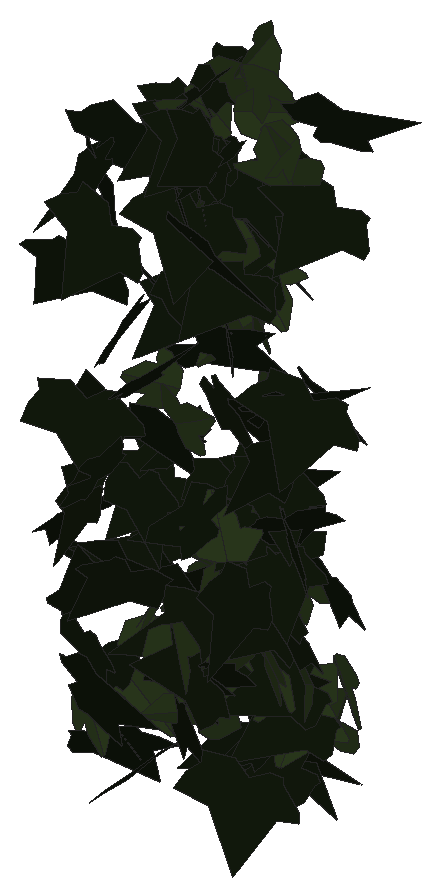
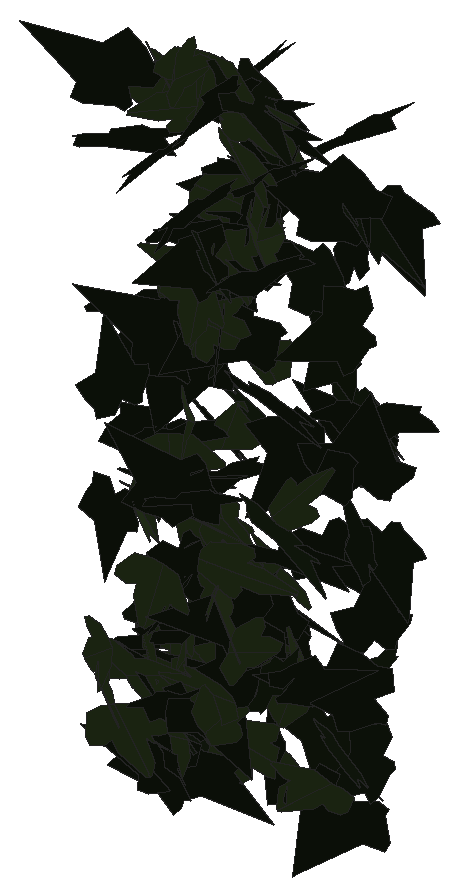
# SketchUp Ruby script. Lengths in inches.
U = 1.inch
M = Sketchup.active_model
def pt(a) = Geom::Point3d.new(a.map { |v| v * U })
def face(e, loops, mat)
  f = e.add_face(loops[0].map { |a| pt(a) })
  loops[1..].each { |l| e.add_face(l.map { |a| pt(a) }).erase! }
  f.material = f.back_material = mat if mat
  f
end
# faces: each face lists its corners as indices into pts; further lists are holes
def faces(e, pts, list, mat = nil) = list.each { |f| face(e, (f[0].is_a?(Array) ? f : [f]).map { |l| l.map { |i| pts[i] } }, mat) }
# xy, xz, yz: faces in a plane at the given z, y or x. An outline is a flat list of corners, or four numbers for a rectangle; further outlines are holes
def ring(l) = l.size == 4 ? [[l[0], l[1]], [l[2], l[1]], [l[2], l[3]], [l[0], l[3]]] : l.each_slice(2).to_a
def flat(e, list, mat, &to3) = list.each { |f| face(e, (f[0].is_a?(Array) ? f : [f]).map { |l| ring(l).map { |u, v| to3.(u, v) } }, mat) }
def xy(e, z, list, mat = nil) = flat(e, list, mat) { |x, y| [x, y, z] }
def xz(e, y, list, mat = nil) = flat(e, list, mat) { |x, z| [x, y, z] }
def yz(e, x, list, mat = nil) = flat(e, list, mat) { |y, z| [x, y, z] }
def lines(e, pts, list) = list.each { |a, b| e.add_line(pt(pts[a]), pt(pts[b])) }
# prism: a flat outline (further loops are holes) pulled along v
def prism(e, loops, v, mat = nil)
  f = face(e, loops, mat); d = Geom::Vector3d.new(v.map { |x| x * U })
  f.pushpull(f.normal.samedirection?(d) ? d.length : -d.length)
end
def box(e, o, s, mat = nil) = prism(e, [[o, [o[0] + s[0], o[1], o[2]], [o[0] + s[0], o[1] + s[1], o[2]], [o[0], o[1] + s[1], o[2]]]], [0, 0, s[2]], mat)
def at(x, y, z, deg = 0) = Geom::Transformation.translation(pt([x, y, z])) * Geom::Transformation.rotation(ORIGIN, Z_AXIS, deg.degrees)
def axes(o, x, y, z) = Geom::Transformation.new([*x, 0, *y, 0, *z, 0, *pt(o).to_a, 1])
def part(name) = M.definitions.add(name)
# library, detail: a bought-in or finely detailed component or shape, given as its bounding box
def library(name, o, s) = part(name).tap { |d| box(d.entities, o, s) }
def detail(e, o, s) = box(e.add_group.entities, o, s)
def put(e, d, t, mat = nil) = e.add_instance(d, t).tap { |i| i.material = mat if mat }
def group(e, t, mat = nil) = e.add_group.tap { |g| g.transformation = t; g.material = mat if mat }.entities
root = M.entities
M.materials.add("1026 AP 7946 SUNNY SIDE UP").color = [254, 231, 186]
M.materials.add("efeu1").color = [18, 25, 13]
M.materials.add("efeu2").color = [43, 57, 29]
c1 = part("ivyleaf_9")
p = [[1.54,2.16,1.25],[1.36,2.04,1.19],[-0.21,0.99,0.68],[-0.71,1.11,0.82],[-0.85,0.86,0.67],[-0.8,0.17,0.21],
  [-0.9,-0.01,0.1],[-0.67,-0.16,-0.02],[-0.08,-0.08,-0.05],[-0.03,-0.6,-0.4],[0.65,-0.88,-0.66],[0.83,-0.6,-0.49],
  [1.29,-0.42,-0.43],[1.8125,-0.07,-0.26],[1.21,0.44,0.15]]
faces(c1.entities,p,[[0,1,2,3,4,5,6,7,8,9,10,11,12,13,14]],"efeu1")
c2 = part("ivyleaf_10")
p = [[0,0.5,-0.03],[-0.0625,2.02,-0.43],[-0.19,2.01,-0.46],[-0.54,1.05,-0.29],[-0.52,0.625,-0.18],[-0.83,0.76,-0.28],
  [-1.16,0.64,-0.33],[-1.15,0.33,-0.24],[-0.77,-0.39,0.02],[-0.3,-0.51,0.16],[0.04,-0.48,0.23],[-0.02,2.01,-0.4375],
  [-0.06,2.01,-0.43],[0.04,-0.49,0.23],[0.67,-0.49,0.14],[1.38,0.36,-0.2],[1.375,0.51,-0.24],[0.81,0.65,-0.19],
  [0.62,0.59,-0.15],[0.6,1.09,-0.28],[0.5,1.23,-0.31]]
faces(c2.entities,p,[[0,1,2,3,4,5,6,7,8,9,10],[11,12,0,13,14,15,16,17,18,19,20]],"efeu2")
put(root,c1,axes([143.12,206.38,282.79],[0.44243,-0.08398,-0.36172],[0.56659,0.04987,0.28587],[-0.01992,-0.4468,0.09716]),"1026 AP 7946 SUNNY SIDE UP")
put(root,c1,axes([142.05,208.34,288.9],[-0.2726,-0.37462,0.23144],[-0.11476,-0.21578,-0.42595],[0.67895,-0.18688,0.02093]),"1026 AP 7946 SUNNY SIDE UP")
put(root,c1,axes([141.82,208.15,284.62],[-0.4204,0.06283,-0.26024],[0.35853,-0.11923,-0.27946],[-0.1986,-0.34823,0.04639]),"1026 AP 7946 SUNNY SIDE UP")
put(root,c1,axes([144.47,208.41,283.86],[-0.56265,0.0144,-0.29484],[0.43446,-0.10455,-0.36181],[-0.11997,-0.44617,0.07251]),"1026 AP 7946 SUNNY SIDE UP")
put(root,c1,axes([141.93,208.21,284.87],[-0.15575,0.37355,0.17332],[-0.08965,0.15663,-0.39696],[-0.63655,-0.11346,0.0135]),"1026 AP 7946 SUNNY SIDE UP")
put(root,c1,axes([141.4375,208.46,288.125],[0.29042,0.15248,-0.34098],[-0.36608,-0.23735,-0.24723],[-0.44243,0.29648,-0.01926]),"1026 AP 7946 SUNNY SIDE UP")
put(root,c1,axes([142.39,208.34,286.4],[0.14354,0.3645,0.012],[-0.01735,-0.00711,0.38695],[0.57307,-0.09152,0.00871]),"1026 AP 7946 SUNNY SIDE UP")
put(root,c1,axes([143.16,209.09,281.73],[0.15178,-0.38666,-0.21939],[0.10483,-0.20045,0.40912],[-0.68446,-0.11644,0.01401]),"1026 AP 7946 SUNNY SIDE UP")
put(root,c2,axes([141.36,208.77,280.88],[0.07741,0.38036,0.01188],[0.01152,0.0085,-0.39501],[-0.59815,0.04939,-0.00607]),"1026 AP 7946 SUNNY SIDE UP")
put(root,c2,axes([142.67,208.95,282.22],[0.46094,-0.0967,0.25303],[0.34219,-0.12062,-0.31651],[0.23631,0.36329,-0.03523]),"1026 AP 7946 SUNNY SIDE UP")
put(root,c1,axes([143.46,208.8,284.49],[-0.48947,0.28617,0.02774],[-0.06477,-0.00754,-0.4343],[-0.44707,-0.31222,0.03255]),"1026 AP 7946 SUNNY SIDE UP")
put(root,c1,axes([141.92,208.96,283],[0.06925,0.16992,-0.33266],[-0.12073,-0.31465,-0.18266],[-0.56229,0.08849,-0.00175]),"1026 AP 7946 SUNNY SIDE UP")
put(root,c1,axes([142.16,208.66,279.99],[0.03692,0.43094,0.13115],[0.02107,0.1243,-0.44383],[-0.70516,0.02628,-0.00639]),"1026 AP 7946 SUNNY SIDE UP")
put(root,c1,axes([141.01,209.15,285.36],[-0.32294,-0.33576,-0.18098],[0.15676,0.14266,-0.40452],[0.57342,-0.22809,0.00866]),"1026 AP 7946 SUNNY SIDE UP")
put(root,c1,axes([141.9,209.24,284.35],[0.03203,-0.384,-0.01787],[-0.0151,0.01467,-0.39596],[0.60408,0.02073,-0.00895]),"1026 AP 7946 SUNNY SIDE UP")
put(root,c1,axes([143.76,209.3125,280.15],[-0.36982,-0.36561,-0.07981],[0.09047,0.05254,-0.44708],[0.57996,-0.24133,0.01885]),"1026 AP 7946 SUNNY SIDE UP")
put(root,c2,axes([143.53,209.05,283.97],[0.32725,0.30847,-0.00686],[-0.02625,0.02138,0.38255],[0.48451,-0.20719,0.02536]),"1026 AP 7946 SUNNY SIDE UP")
put(root,c1,axes([140.79,209.375,281.43],[0.10485,-0.31947,0.16809],[0.06172,-0.16032,-0.3371],[0.56198,0.07721,0.00566]),"1026 AP 7946 SUNNY SIDE UP")
put(root,c1,axes([142.92,209.51,289.92],[-0.19153,-0.22079,0.35133],[-0.18402,-0.32322,-0.25959],[0.61346,-0.1659,0.03182]),"1026 AP 7946 SUNNY SIDE UP")
put(root,c2,axes([142.61,209.26,285.53],[-0.36477,0.08808,0.28437],[0.42651,-0.05647,0.25354],[0.15803,0.35573,-0.0279]),"1026 AP 7946 SUNNY SIDE UP")
put(root,c1,axes([140.79,209.32,282.06],[0.24725,0.21741,0.2574],[-0.33171,-0.14575,0.26791],[0.39958,-0.25553,0.06313]),"1026 AP 7946 SUNNY SIDE UP")
put(root,c1,axes([142.94,209.125,281.74],[0.32619,0.30069,-0.13353],[-0.09417,-0.11806,-0.37663],[-0.50726,0.21527,-0.01595]),"1026 AP 7946 SUNNY SIDE UP")
put(root,c1,axes([144.12,209.53,285.39],[-0.0119,-0.01258,-0.38765],[0.23781,-0.34469,0.00672],[-0.54203,-0.15095,0.01146]),"1026 AP 7946 SUNNY SIDE UP")
put(root,c1,axes([140.78,209.16,283.52],[-0.00412,0.35045,-0.0916],[0.00426,-0.09088,-0.36156],[-0.56926,-0.00322,-0.00205]),"1026 AP 7946 SUNNY SIDE UP")
put(root,c1,axes([142.98,209.5,282.25],[-0.64066,0.07545,0.10485],[-0.16802,-0.02314,-0.42492],[-0.10603,-0.41922,0.03979]),"1026 AP 7946 SUNNY SIDE UP")
put(root,c1,axes([142.44,209.3,281.54],[0.55431,0.08529,-0.08372],[-0.11064,-0.05507,-0.37211],[-0.14922,0.35766,-0.03508]),"1026 AP 7946 SUNNY SIDE UP")
put(root,c1,axes([142.49,209.51,288.375],[0.47747,-0.19271,0.19285],[0.2198,-0.12984,-0.36991],[0.36217,0.33287,-0.02975]),"1026 AP 7946 SUNNY SIDE UP")
put(root,c1,axes([142.52,209.7,288.73],[-0.51922,-0.2567,-0.15212],[0.21609,0.06063,-0.42906],[0.41119,-0.356,0.03339]),"1026 AP 7946 SUNNY SIDE UP")
put(root,c1,axes([142.98,209.62,285.99],[0.38973,-0.31497,-0.06263],[-0.08538,0.03224,-0.41206],[0.49659,0.25274,-0.0217]),"1026 AP 7946 SUNNY SIDE UP")
put(root,c2,axes([143.28,209.88,281.94],[0.00507,-0.03015,0.38475],[0.03999,-0.37278,-0.03339],[0.58807,0.02561,-0.00105]),"1026 AP 7946 SUNNY SIDE UP")
put(root,c1,axes([140.73,209.7,284.63],[0.46765,0.11317,0.24676],[-0.37638,-0.03727,0.32498],[0.17634,-0.37965,0.03922]),"1026 AP 7946 SUNNY SIDE UP")
put(root,c1,axes([143.21,209.86,287.86],[-0.53292,-0.23031,0.03867],[-0.01345,-0.05617,-0.4203],[0.36701,-0.33648,0.04075]),"1026 AP 7946 SUNNY SIDE UP")
put(root,c1,axes([140.79,209.73,288.89],[-0.51202,0.23851,-0.23296],[0.24214,-0.17264,-0.41457],[-0.45822,-0.35774,0.04124]),"1026 AP 7946 SUNNY SIDE UP")
put(root,c1,axes([144.45,209.88,286.22],[-0.41158,-0.35677,-0.01094],[0.04568,-0.01068,-0.45489],[0.55929,-0.26168,0.0291]),"1026 AP 7946 SUNNY SIDE UP")
put(root,c1,axes([142.57,209.91,289.81],[-0.44555,-0.25057,0.10766],[-0.09453,-0.0915,-0.38917],[0.41719,-0.28834,0.0268]),"1026 AP 7946 SUNNY SIDE UP")
put(root,c1,axes([143,209.53,289.67],[-0.27285,0.38439,0.03783],[-0.06804,0.01825,-0.43313],[-0.60303,-0.17599,0.03175]),"1026 AP 7946 SUNNY SIDE UP")
put(root,c1,axes([143.83,209.86,283.53],[-0.33167,-0.26346,-0.20986],[0.39525,0.02992,-0.3101],[0.3413,-0.29067,0.15518]),"1026 AP 7946 SUNNY SIDE UP")
put(root,c1,axes([140.39,209.71,280.51],[0.54395,-0.22368,-0.06371],[-0.10307,0.00995,-0.42342],[0.34951,0.35106,-0.0257]),"1026 AP 7946 SUNNY SIDE UP")
put(root,c2,axes([143.05,209.95,288.33],[-0.22242,-0.05886,0.3503],[-0.32832,-0.27843,-0.14063],[0.43267,-0.24153,0.07337]),"1026 AP 7946 SUNNY SIDE UP")
put(root,c1,axes([144.28,209.61,284.14],[0.35956,-0.12418,-0.34885],[-0.47179,0.1555,-0.26713],[0.31284,0.37723,-0.00191]),"1026 AP 7946 SUNNY SIDE UP")
put(root,c2,axes([143.31,209.79,283.14],[-0.47872,0.00758,0.25202],[-0.37642,-0.09017,-0.30463],[0.07977,-0.37998,0.07497]),"1026 AP 7946 SUNNY SIDE UP")
put(root,c1,axes([141.33,209.43,286.45],[-0.17226,0.17161,-0.37816],[-0.35854,0.28945,0.21065],[0.52839,0.25235,0.01965]),"1026 AP 7946 SUNNY SIDE UP")
put(root,c1,axes([140.58,210.04,288.2],[-0.08294,0.02046,0.46293],[0.06695,-0.45007,0.02363],[0.70395,0.04521,0.05229]),"1026 AP 7946 SUNNY SIDE UP")
put(root,c1,axes([142.3,209.98,289.8],[-0.6167,-0.05032,0.01399],[-0.01354,-0.04125,-0.40553],[0.08094,-0.39027,0.03871]),"1026 AP 7946 SUNNY SIDE UP")
put(root,c2,axes([143.18,209.79,283.33],[-0.24214,0.05065,0.35631],[-0.54177,0.03988,-0.16396],[-0.09002,-0.37623,0.02832]),"1026 AP 7946 SUNNY SIDE UP")
put(root,c1,axes([140.44,209.94,283.625],[0.03511,0.2831,0.24296],[-0.0836,-0.2297,0.28989],[0.57168,-0.05098,0.02747]),"1026 AP 7946 SUNNY SIDE UP")
put(root,c1,axes([141.96,210.02,282.03],[0.12206,-0.04175,0.41688],[0.45685,-0.28301,-0.0891],[0.44826,0.2998,-0.0227]),"1026 AP 7946 SUNNY SIDE UP")
put(root,c1,axes([143.66,210.22,282.41],[0.08099,-0.12299,-0.37178],[0.22733,-0.3299,0.13541],[-0.5536,-0.15346,0.00122]),"1026 AP 7946 SUNNY SIDE UP")
put(root,c1,axes([144.08,209.77,284.27],[0.22683,0.37035,-0.06437],[-0.02161,-0.06394,-0.40969],[-0.59073,0.14455,-0.00973]),"1026 AP 7946 SUNNY SIDE UP")
put(root,c1,axes([143.4,210.25,283.89],[-0.40474,-0.26229,0.1372],[-0.04005,-0.15832,-0.36874],[0.46188,-0.24357,0.08825]),"1026 AP 7946 SUNNY SIDE UP")
put(root,c1,axes([140.85,209.76,279.66],[0.51591,0.2461,0.00876],[0.03373,-0.01678,-0.42176],[-0.38567,0.32775,-0.02517]),"1026 AP 7946 SUNNY SIDE UP")
put(root,c1,axes([142.18,209.91,288.49],[0.06993,-0.30014,0.31427],[0.01279,0.30894,0.31199],[-0.67471,-0.02525,0.03849]),"1026 AP 7946 SUNNY SIDE UP")
put(root,c2,axes([141.92,210.24,288.13],[0.09879,-0.10183,0.35885],[0.23826,-0.31451,-0.12451],[0.51949,0.16362,-0.01113]),"1026 AP 7946 SUNNY SIDE UP")
put(root,c1,axes([142.36,209.73,287.69],[0.13713,-0.07715,-0.43675],[-0.04406,0.43019,-0.08416],[0.67546,0.04372,0.08318]),"1026 AP 7946 SUNNY SIDE UP")
put(root,c1,axes([141.3,209.85,284.95],[0.67688,0.08147,-0.02386],[-0.02483,-0.04309,-0.44978],[-0.13105,0.42897,-0.03803]),"1026 AP 7946 SUNNY SIDE UP")
put(root,c1,axes([144.1,210.22,280.97],[-0.55806,-0.163,0.08858],[-0.08096,-0.09348,-0.3978],[0.27895,-0.35323,0.06175]),"1026 AP 7946 SUNNY SIDE UP")
put(root,c2,axes([142.12,210.21,288.29],[0.21091,-0.27944,0.25574],[0.20815,-0.21294,-0.31983],[0.55143,0.18726,0.02291]),"1026 AP 7946 SUNNY SIDE UP")
put(root,c2,axes([143.36,210.08,281.44],[0.56879,0.00039,-0.14059],[-0.21332,-0.04096,-0.37081],[-0.02331,0.38444,-0.03709]),"1026 AP 7946 SUNNY SIDE UP")
put(root,c1,axes([143.59,209.89,285.78],[0.52195,0.22022,-0.12229],[-0.13209,-0.08986,-0.40994],[-0.37153,0.34133,-0.02606]),"1026 AP 7946 SUNNY SIDE UP")
put(root,c1,axes([143.96,210.29,281.38],[-0.46694,-0.16254,0.21107],[-0.2466,-0.13914,-0.34713],[0.33051,-0.33344,0.03921]),"1026 AP 7946 SUNNY SIDE UP")
put(root,c1,axes([143.66,209.85,285.83],[0.30116,0.33812,-0.16313],[0.10228,0.14722,0.4009],[0.5794,-0.20173,0.01402]),"1026 AP 7946 SUNNY SIDE UP")
put(root,c2,axes([143.87,210.0625,290.125],[0.3835,-0.26763,-0.10511],[-0.13896,0.05506,-0.37165],[0.42751,0.25798,-0.02652]),"1026 AP 7946 SUNNY SIDE UP")
put(root,c2,axes([143.86,210.11,289.61],[-0.51483,-0.13838,-0.12449],[-0.19589,-0.01209,0.3643],[-0.21121,0.34852,-0.03443]),"1026 AP 7946 SUNNY SIDE UP")
put(root,c1,axes([140.89,210.16,280.76],[-0.45103,0.12532,-0.16941],[0.20492,-0.11029,-0.32003],[-0.25354,-0.31208,0.04273]),"1026 AP 7946 SUNNY SIDE UP")
put(root,c1,axes([142.51,210.01,288.07],[0.10898,-0.24415,0.27117],[0.04734,0.27245,0.25245],[-0.56414,-0.0243,0.07357]),"1026 AP 7946 SUNNY SIDE UP")
put(root,c1,axes([143.57,210.19,284.61],[-0.16818,-0.36023,-0.12294],[0.06469,0.11011,-0.38639],[0.59217,-0.11434,0.00729]),"1026 AP 7946 SUNNY SIDE UP")
put(root,c1,axes([142.77,210.22,284.27],[-0.11185,-0.38103,-0.09045],[0.02189,0.08452,-0.39882],[0.61369,-0.07246,-0.00226]),"1026 AP 7946 SUNNY SIDE UP")
put(root,c1,axes([141.66,210.29,280.25],[0.1325,-0.09853,-0.41191],[0.62414,-0.08714,0.10794],[-0.16918,-0.39866,0.07562]),"1026 AP 7946 SUNNY SIDE UP")
put(root,c1,axes([142.5625,209.8125,286.55],[0.49347,0.26703,0.17183],[0.23146,0.08133,-0.42282],[-0.4362,0.34525,-0.02996]),"1026 AP 7946 SUNNY SIDE UP")
put(root,c2,axes([141.24,210.18,281.47],[0.17156,-0.35402,-0.09988],[0.08752,-0.08191,0.38006],[-0.56965,-0.1192,0.02831]),"1026 AP 7946 SUNNY SIDE UP")
put(root,c1,axes([144.01,210.125,283.43],[-0.49233,0.22223,0.19155],[-0.36317,-0.02886,-0.3678],[-0.27301,-0.36236,0.14383]),"1026 AP 7946 SUNNY SIDE UP")
put(root,c1,axes([143.45,210.15,282.77],[-0.13368,0.29831,-0.23591],[0.09894,-0.22194,-0.32085],[-0.58465,-0.10577,-0.00036]),"1026 AP 7946 SUNNY SIDE UP")
put(root,c2,axes([142.25,210.18,289.87],[0.42241,0.0334,-0.25489],[-0.39024,-0.00632,-0.2783],[-0.04537,0.36529,0.02065]),"1026 AP 7946 SUNNY SIDE UP")
put(root,c2,axes([141.5,210.13,281.41],[0.5209,0.18083,0.09088],[0.11874,0.04364,-0.38855],[-0.29249,0.33977,0.00412]),"1026 AP 7946 SUNNY SIDE UP")
put(root,c2,axes([143.96,210.26,280.94],[0.46804,0.24245,-0.12189],[-0.11407,-0.09988,-0.39486],[-0.40957,0.30488,-0.02932]),"1026 AP 7946 SUNNY SIDE UP")
put(root,c2,axes([142.78,210.46,286.65],[-0.14189,-0.1953,0.33702],[-0.04032,-0.33343,-0.21358],[0.59924,-0.06868,0.06543]),"1026 AP 7946 SUNNY SIDE UP")
put(root,c1,axes([143.65,210.48,282.03],[-0.05734,-0.22505,0.3055],[0.11562,-0.29771,-0.22422],[0.57547,0.03739,0.07549]),"1026 AP 7946 SUNNY SIDE UP")
put(root,c1,axes([140.55,210.14,288.97],[0.16748,-0.00364,0.43429],[0.64684,-0.09427,-0.10846],[0.14509,0.42448,-0.01776]),"1026 AP 7946 SUNNY SIDE UP")
put(root,c1,axes([142.8,210.0625,286.91],[0.228,-0.12818,-0.36006],[-0.49027,0.1617,-0.19381],[0.31786,0.34136,-0.04067]),"1026 AP 7946 SUNNY SIDE UP")
put(root,c1,axes([144.34,210.51,289.04],[-0.48159,-0.29258,0.09811],[-0.04396,-0.10967,-0.43282],[0.48263,-0.30194,0.05848]),"1026 AP 7946 SUNNY SIDE UP")
put(root,c2,axes([143.49,210.12,281.57],[-0.33812,0.27692,0.15472],[-0.24116,0.06471,-0.35245],[-0.43132,-0.25326,0.07577]),"1026 AP 7946 SUNNY SIDE UP")
put(root,c1,axes([143.09,210.5,281.84],[-0.43248,-0.28157,0.08686],[-0.05161,-0.08751,-0.40423],[0.46001,-0.27454,0.03631]),"1026 AP 7946 SUNNY SIDE UP")
put(root,c2,axes([143.53,210.28,284.37],[-0.37473,-0.3237,-0.00074],[0.02825,-0.01461,-0.4135],[0.5082,-0.23787,0.02244]),"1026 AP 7946 SUNNY SIDE UP")
put(root,c2,axes([143.36,210.2,281.73],[-0.39629,0.26581,0.02718],[-0.05502,0.00103,-0.3765],[-0.41617,-0.25325,0.02389]),"1026 AP 7946 SUNNY SIDE UP")
put(root,c2,axes([142.31,210.38,280.35],[-0.24645,-0.05772,0.37905],[-0.48946,-0.19951,-0.16986],[0.32246,-0.34695,0.03186]),"1026 AP 7946 SUNNY SIDE UP")
put(root,c1,axes([143.43,210.3,280.38],[-0.4709,0.24682,-0.0901],[0.07733,-0.07964,-0.39911],[-0.40517,-0.30206,0.02854]),"1026 AP 7946 SUNNY SIDE UP")
put(root,c1,axes([141.41,210.53,283.66],[-0.54813,-0.18847,0.02821],[-0.01404,-0.0431,-0.40703],[0.29939,-0.34709,0.03256]),"1026 AP 7946 SUNNY SIDE UP")
put(root,c1,axes([142.37,210.22,290.5],[-0.25654,0.38976,-0.0528],[-0.00004,-0.05789,-0.43502],[-0.6186,-0.16164,0.02192]),"1026 AP 7946 SUNNY SIDE UP")
put(root,c1,axes([143.38,210.63,282.05],[-0.10148,-0.15829,0.33795],[-0.16789,-0.31125,-0.1777],[0.54889,-0.12447,0.00812]),"1026 AP 7946 SUNNY SIDE UP")
put(root,c1,axes([142.76,210.53,287.59],[-0.55462,-0.20896,-0.03588],[0.06281,-0.00151,-0.42177],[0.32682,-0.35432,0.02016]),"1026 AP 7946 SUNNY SIDE UP")
put(root,c1,axes([144.53,210.24,283.27],[0.40436,-0.04837,-0.27473],[-0.41915,0.01918,-0.26856],[0.07463,0.36978,-0.0198]),"1026 AP 7946 SUNNY SIDE UP")
put(root,c2,axes([144.09,210.18,281.47],[0.21949,-0.17452,-0.34205],[-0.21405,0.30542,-0.22323],[0.54811,0.18916,0.04979]),"1026 AP 7946 SUNNY SIDE UP")
put(root,c2,axes([142.875,210.08,287.14],[-0.07238,0.11483,0.3915],[-0.2828,0.33429,-0.12476],[-0.5554,-0.18518,0.01251]),"1026 AP 7946 SUNNY SIDE UP")
put(root,c1,axes([140.23,210.38,287.47],[0.58747,-0.2219,0.01737],[0.01114,-0.02353,-0.44747],[0.3499,0.37331,-0.01492]),"1026 AP 7946 SUNNY SIDE UP")
put(root,c1,axes([143.73,210.48,279.85],[-0.52835,0.04642,0.04673],[-0.07714,-0.02712,-0.34792],[-0.06639,-0.33794,0.03232]),"1026 AP 7946 SUNNY SIDE UP")
put(root,c1,axes([141.95,210.45,281.4],[0.41056,0.2533,0.13833],[-0.17856,-0.07328,0.37346],[0.41277,-0.28364,0.02396]),"1026 AP 7946 SUNNY SIDE UP")
put(root,c2,axes([142.29,210.53,288.03],[-0.06764,-0.38171,0.06288],[-0.00239,-0.06342,-0.39605],[0.60837,-0.04269,0.00544]),"1026 AP 7946 SUNNY SIDE UP")
put(root,c2,axes([140.8,210.43,280.21],[0.38996,0.13713,0.23163],[0.32495,0.08838,-0.29086],[-0.255,0.32233,-0.01643]),"1026 AP 7946 SUNNY SIDE UP")
put(root,c1,axes([140.03,210.39,281.85],[0.34119,0.02689,0.32871],[0.50308,-0.02864,-0.22193],[0.0136,0.38468,-0.03723]),"1026 AP 7946 SUNNY SIDE UP")
put(root,c1,axes([142.91,210.62,279.9],[0.05008,0.02527,-0.36038],[-0.31042,-0.28922,-0.04171],[-0.45611,0.19961,-0.01118]),"1026 AP 7946 SUNNY SIDE UP")
put(root,c1,axes([141.59,210.83,289.42],[-0.30811,-0.25769,0.23555],[-0.14713,-0.21507,-0.33146],[0.52292,-0.21234,0.04553]),"1026 AP 7946 SUNNY SIDE UP")
put(root,c2,axes([143.0625,210.375,286.96],[-0.32012,0.23634,0.21718],[-0.25997,0.13258,-0.31887],[-0.42309,-0.26029,0.0316]),"1026 AP 7946 SUNNY SIDE UP")
put(root,c2,axes([143.72,210.7,283.71],[0.2129,-0.31334,0.15058],[0.09242,-0.13577,-0.35244],[0.53696,0.14761,0.00096]),"1026 AP 7946 SUNNY SIDE UP")
put(root,c2,axes([142.75,210.54,290.64],[-0.61533,-0.05719,-0.02767],[0.05009,-0.03537,-0.4056],[0.08555,-0.39063,0.03843]),"1026 AP 7946 SUNNY SIDE UP")
put(root,c2,axes([141.93,210.81,282.09],[0.0969,0.11392,-0.38348],[-0.26527,-0.33256,-0.13534],[-0.55273,0.17958,-0.00228]),"1026 AP 7946 SUNNY SIDE UP")
put(root,c1,axes([142.85,210.79,288.23],[-0.33123,-0.31023,0.02544],[0.00403,-0.03367,-0.3859],[0.48956,-0.20962,0.02039]),"1026 AP 7946 SUNNY SIDE UP")
put(root,c2,axes([142.85,210.55,287.54],[0.49149,0.15537,0.20192],[0.30319,0.04792,-0.35724],[-0.24878,0.36535,-0.03645]),"1026 AP 7946 SUNNY SIDE UP")
put(root,c1,axes([142.03,210.28,282.28],[0.09337,0.25214,-0.33159],[0.09319,0.31796,0.26854],[0.63791,-0.08336,0.0093]),"1026 AP 7946 SUNNY SIDE UP")
put(root,c2,axes([142.56,210.6,282.79],[-0.29131,0.31418,-0.04338],[0.01055,-0.04694,-0.37557],[-0.49871,-0.18452,0.0174]),"1026 AP 7946 SUNNY SIDE UP")
put(root,c1,axes([142.93,210.85,284.08],[-0.37944,-0.28603,0.03135],[-0.00198,-0.04079,-0.38489],[0.45257,-0.23999,0.0246]),"1026 AP 7946 SUNNY SIDE UP")
put(root,c1,axes([142.63,210.74,280.79],[0.04691,0.02483,0.40455],[0.48004,-0.2497,-0.00909],[0.39,0.30437,-0.03747]),"1026 AP 7946 SUNNY SIDE UP")
put(root,c1,axes([142.49,210.84,288.02],[-0.39297,0.09097,-0.23526],[0.27162,-0.1677,-0.26396],[-0.27606,-0.29449,0.07519]),"1026 AP 7946 SUNNY SIDE UP")
put(root,c1,axes([142.59,210.68,281.12],[0.02524,0.3051,-0.23044],[-0.04672,-0.22392,-0.31571],[-0.59465,0.03054,0.01502]),"1026 AP 7946 SUNNY SIDE UP")
put(root,c1,axes([141.21,210.97,281.77],[0.02098,-0.23229,0.28886],[0.05911,-0.27953,-0.24092],[0.57108,0.03747,0.01433]),"1026 AP 7946 SUNNY SIDE UP")
put(root,c1,axes([143.08,210.77,279.89],[0.2898,-0.10937,0.30951],[0.39605,-0.16511,-0.2216],[0.31116,0.312,-0.00621]),"1026 AP 7946 SUNNY SIDE UP")
put(root,c2,axes([142.23,210.97,280.96],[-0.11605,-0.1674,-0.35828],[-0.2593,-0.30539,0.18621],[-0.54723,0.18021,-0.01226]),"1026 AP 7946 SUNNY SIDE UP")
put(root,c2,axes([142.91,210.88,280.43],[-0.23857,0.10054,-0.31204],[0.24672,-0.26925,-0.17428],[-0.43796,-0.20644,0.07179]),"1026 AP 7946 SUNNY SIDE UP")
put(root,c1,axes([142.96,210.67,284.06],[0.49023,0.14891,-0.11104],[0.11357,0.09769,0.35207],[0.26665,-0.31537,0.0542]),"1026 AP 7946 SUNNY SIDE UP")
put(root,c2,axes([142.28,210.77,283.27],[0.1259,-0.04761,-0.37906],[-0.5828,-0.00104,-0.08302],[0.01432,0.3763,-0.04595]),"1026 AP 7946 SUNNY SIDE UP")
put(root,c2,axes([143.8,210.67,280.96],[0.39926,0.04592,0.31931],[-0.49148,0.01438,0.2619],[0.02816,-0.40022,0.04367]),"1026 AP 7946 SUNNY SIDE UP")
put(root,c2,axes([141.93,210.8,289.76],[0.52183,-0.21418,-0.02628],[-0.06175,-0.01622,-0.40541],[0.33327,0.33236,-0.03397]),"1026 AP 7946 SUNNY SIDE UP")
put(root,c1,axes([140.9,210.97,281.94],[-0.20707,-0.0453,0.35475],[-0.47802,-0.16363,-0.1428],[0.26494,-0.33064,0.01963]),"1026 AP 7946 SUNNY SIDE UP")
put(root,c1,axes([142.19,210.58,290.54],[0.17623,-0.15682,-0.3235],[-0.16296,0.2992,-0.19083],[0.526,0.14524,0.04926]),"1026 AP 7946 SUNNY SIDE UP")
put(root,c2,axes([142.73,210.73,287.3],[-0.54507,0.16979,0.0245],[-0.05533,-0.02017,-0.39627],[-0.26363,-0.34681,0.03251]),"1026 AP 7946 SUNNY SIDE UP")
put(root,c1,axes([141.48,210.96,288.13],[-0.12587,-0.41074,-0.0409],[0.03457,0.03376,-0.43062],[0.64759,-0.08164,0.01504]),"1026 AP 7946 SUNNY SIDE UP")
put(root,c1,axes([143.25,210.81,289.3],[0.16427,-0.33186,-0.14086],[-0.05344,0.13065,-0.3576],[0.56072,0.10968,0.00719]),"1026 AP 7946 SUNNY SIDE UP")
put(root,c1,axes([142.56,210.82,288.77],[0.16508,-0.3685,-0.17222],[-0.07897,0.15733,-0.39378],[0.62998,0.11628,-0.00424]),"1026 AP 7946 SUNNY SIDE UP")
put(root,c2,axes([144.18,210.92,281.375],[-0.23871,0.21402,-0.27739],[0.19859,-0.2405,-0.27048],[-0.50468,-0.19587,0.02477]),"1026 AP 7946 SUNNY SIDE UP")
put(root,c1,axes([143.1875,210.89,279.89],[-0.05923,-0.06907,-0.37548],[0.57355,0.0577,-0.04982],[0.10288,-0.36145,0.06155]),"1026 AP 7946 SUNNY SIDE UP")
put(root,c2,axes([144.125,210.95,280.82],[0.27845,-0.29064,0.14565],[0.11683,-0.12222,-0.35133],[0.49577,0.19204,0.00098]),"1026 AP 7946 SUNNY SIDE UP")
put(root,c2,axes([142.19,210.85,282.66],[0.22299,-0.32948,-0.01237],[-0.02279,0.0048,-0.36932],[0.51782,0.14209,-0.01093]),"1026 AP 7946 SUNNY SIDE UP")
put(root,c2,axes([142.86,210.57,290.04],[0.00159,0.01116,0.38902],[0.19339,0.35697,-0.00912],[-0.56156,0.12296,-0.00204]),"1026 AP 7946 SUNNY SIDE UP")
put(root,c2,axes([143.35,210.81,282.73],[-0.57427,0.11734,-0.02012],[0.01534,-0.03544,-0.39412],[-0.18658,-0.36405,0.02951]),"1026 AP 7946 SUNNY SIDE UP")
put(root,c1,axes([143.91,210.79,290.11],[0.11377,-0.08368,0.38799],[0.59787,-0.05217,-0.08739],[0.10701,0.38041,0.07574]),"1026 AP 7946 SUNNY SIDE UP")
put(root,c1,axes([141.43,210.64,284.12],[-0.14473,0.3394,0.20306],[-0.21801,0.15925,-0.35171],[-0.57573,-0.14562,0.08214]),"1026 AP 7946 SUNNY SIDE UP")
put(root,c2,axes([140.875,211.08,284.75],[-0.00724,0.20746,0.34196],[0.02176,-0.33049,0.21181],[0.61354,0.01417,-0.00348]),"1026 AP 7946 SUNNY SIDE UP")
put(root,c1,axes([142.81,210.96,281.14],[-0.12029,-0.33977,-0.1494],[0.1034,0.13122,-0.35645],[0.57041,-0.09544,0.03311]),"1026 AP 7946 SUNNY SIDE UP")
put(root,c2,axes([143.88,210.92,280.39],[-0.47958,-0.14406,0.16034],[-0.19954,-0.09624,-0.3467],[0.26836,-0.329,0.02875]),"1026 AP 7946 SUNNY SIDE UP")
put(root,c1,axes([142.33,210.89,288.04],[0.54997,-0.20386,0.04273],[0.03595,-0.04524,-0.41637],[0.32551,0.34944,-0.0262]),"1026 AP 7946 SUNNY SIDE UP")
put(root,c2,axes([142.67,211.15,290.84],[0.05437,0.10032,-0.38934],[-0.11487,-0.37165,-0.11053],[-0.60489,0.0796,-0.014]),"1026 AP 7946 SUNNY SIDE UP")
put(root,c2,axes([142.63,211.08,285.52],[-0.14223,0.19069,-0.30919],[0.03537,-0.30708,-0.20903],[-0.55944,-0.06789,0.06539]),"1026 AP 7946 SUNNY SIDE UP")
put(root,c2,axes([142.17,210.96,281.34],[-0.10786,-0.05227,-0.35324],[0.50064,-0.14739,-0.04337],[-0.21515,-0.31677,0.07616]),"1026 AP 7946 SUNNY SIDE UP")
put(root,c1,axes([141.48,211.03,286.35],[-0.60481,-0.0035,-0.08648],[0.13159,-0.04989,-0.39327],[-0.01139,-0.39051,0.04869]),"1026 AP 7946 SUNNY SIDE UP")
put(root,c1,axes([143.75,211.07,285.49],[0.48458,-0.16854,-0.12605],[0.19833,-0.02073,0.35938],[-0.2595,-0.33058,0.03928]),"1026 AP 7946 SUNNY SIDE UP")
